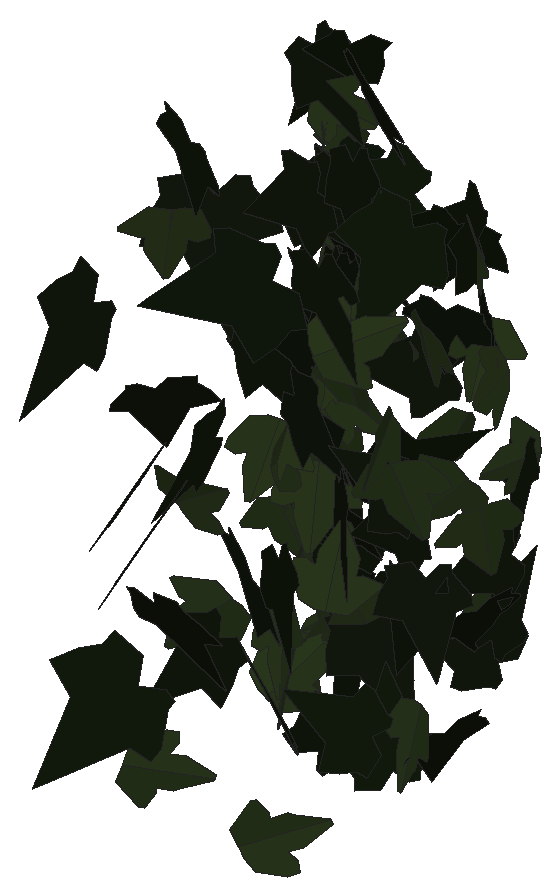
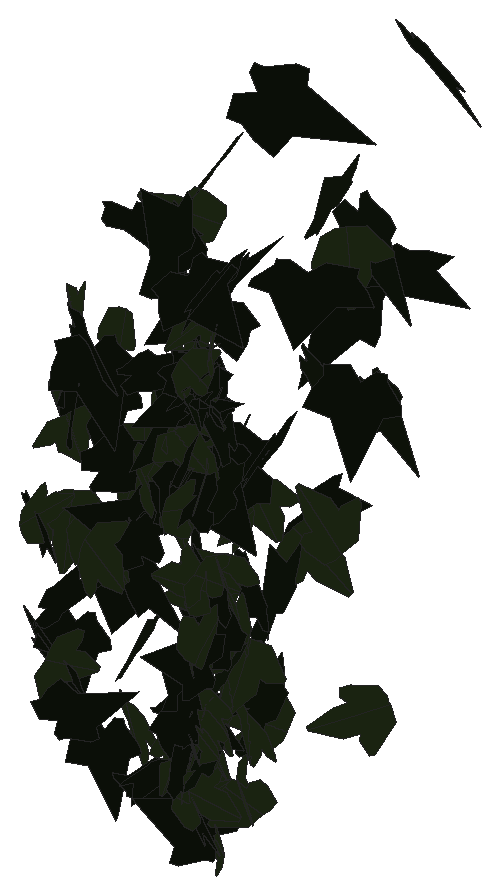
# SketchUp Ruby script. Lengths in inches.
U = 1.inch
M = Sketchup.active_model
def pt(a) = Geom::Point3d.new(a.map { |v| v * U })
def face(e, loops, mat)
  f = e.add_face(loops[0].map { |a| pt(a) })
  loops[1..].each { |l| e.add_face(l.map { |a| pt(a) }).erase! }
  f.material = f.back_material = mat if mat
  f
end
# faces: each face lists its corners as indices into pts; further lists are holes
def faces(e, pts, list, mat = nil) = list.each { |f| face(e, (f[0].is_a?(Array) ? f : [f]).map { |l| l.map { |i| pts[i] } }, mat) }
# xy, xz, yz: faces in a plane at the given z, y or x. An outline is a flat list of corners, or four numbers for a rectangle; further outlines are holes
def ring(l) = l.size == 4 ? [[l[0], l[1]], [l[2], l[1]], [l[2], l[3]], [l[0], l[3]]] : l.each_slice(2).to_a
def flat(e, list, mat, &to3) = list.each { |f| face(e, (f[0].is_a?(Array) ? f : [f]).map { |l| ring(l).map { |u, v| to3.(u, v) } }, mat) }
def xy(e, z, list, mat = nil) = flat(e, list, mat) { |x, y| [x, y, z] }
def xz(e, y, list, mat = nil) = flat(e, list, mat) { |x, z| [x, y, z] }
def yz(e, x, list, mat = nil) = flat(e, list, mat) { |y, z| [x, y, z] }
def lines(e, pts, list) = list.each { |a, b| e.add_line(pt(pts[a]), pt(pts[b])) }
# prism: a flat outline (further loops are holes) pulled along v
def prism(e, loops, v, mat = nil)
  f = face(e, loops, mat); d = Geom::Vector3d.new(v.map { |x| x * U })
  f.pushpull(f.normal.samedirection?(d) ? d.length : -d.length)
end
def box(e, o, s, mat = nil) = prism(e, [[o, [o[0] + s[0], o[1], o[2]], [o[0] + s[0], o[1] + s[1], o[2]], [o[0], o[1] + s[1], o[2]]]], [0, 0, s[2]], mat)
def at(x, y, z, deg = 0) = Geom::Transformation.translation(pt([x, y, z])) * Geom::Transformation.rotation(ORIGIN, Z_AXIS, deg.degrees)
def axes(o, x, y, z) = Geom::Transformation.new([*x, 0, *y, 0, *z, 0, *pt(o).to_a, 1])
def part(name) = M.definitions.add(name)
# library, detail: a bought-in or finely detailed component or shape, given as its bounding box
def library(name, o, s) = part(name).tap { |d| box(d.entities, o, s) }
def detail(e, o, s) = box(e.add_group.entities, o, s)
def put(e, d, t, mat = nil) = e.add_instance(d, t).tap { |i| i.material = mat if mat }
def group(e, t, mat = nil) = e.add_group.tap { |g| g.transformation = t; g.material = mat if mat }.entities
root = M.entities
M.materials.add("efeu1").color = [18, 25, 13]
M.materials.add("efeu2").color = [43, 57, 29]
c1 = part("ivyleaf_9")
p = [[1.54,2.16,1.25],[1.36,2.04,1.19],[-0.21,0.99,0.68],[-0.71,1.11,0.82],[-0.85,0.86,0.67],[-0.8,0.17,0.21],
  [-0.9,-0.01,0.1],[-0.67,-0.16,-0.02],[-0.08,-0.08,-0.05],[-0.03,-0.6,-0.4],[0.65,-0.88,-0.66],[0.83,-0.6,-0.49],
  [1.29,-0.42,-0.43],[1.8125,-0.07,-0.26],[1.21,0.44,0.15]]
faces(c1.entities,p,[[0,1,2,3,4,5,6,7,8,9,10,11,12,13,14]],"efeu1")
c2 = part("ivyleaf_10")
p = [[0,0.5,-0.03],[-0.0625,2.02,-0.43],[-0.19,2.01,-0.46],[-0.54,1.05,-0.29],[-0.52,0.625,-0.18],[-0.83,0.76,-0.28],
  [-1.16,0.64,-0.33],[-1.15,0.33,-0.24],[-0.77,-0.39,0.02],[-0.3,-0.51,0.16],[0.04,-0.48,0.23],[-0.02,2.01,-0.4375],
  [-0.06,2.01,-0.43],[0.04,-0.49,0.23],[0.67,-0.49,0.14],[1.38,0.36,-0.2],[1.375,0.51,-0.24],[0.81,0.65,-0.19],
  [0.62,0.59,-0.15],[0.6,1.09,-0.28],[0.5,1.23,-0.31]]
faces(c2.entities,p,[[0,1,2,3,4,5,6,7,8,9,10],[11,12,0,13,14,15,16,17,18,19,20]],"efeu2")
put(root,c1,axes([593.49,106.23,195.84],[-1.19676,-0.85692,0.36484],[-0.30418,-0.20185,-1.47187],[0.88028,-1.23475,-0.01259]))
put(root,c1,axes([589.84,108.61,207.26],[-1.40402,0.10789,-0.47473],[0.46937,-0.0846,-1.40741],[-0.12921,-1.47969,0.04586]))
put(root,c1,axes([591.91,109.31,199.78],[-0.82844,1.1156,-0.43445],[0.25901,-0.3488,-1.38956],[-1.16885,-0.86799,0.00001]))
put(root,c1,axes([591.93,109.45,196.84],[1.36698,0.20054,-0.333],[-0.32963,-0.04725,-1.38161],[-0.20603,1.40616,0.00107]))
put(root,c1,axes([592.55,114.11,206.7],[-0.2824,-0.17863,-1.47318],[-0.89101,-1.17881,0.31374],[-1.1867,0.92759,0.11501]))
put(root,c1,axes([586.71,115.08,197.1],[-0.73872,0.86965,-0.39727],[0.23479,-0.32165,-1.14071],[-0.92681,-0.77464,0.02766]))
put(root,c1,axes([589.03,115.98,191.73],[0.11357,-0.29781,-1.14485],[0.41787,-1.06587,0.31872],[-1.10669,-0.43302,0.00285]))
put(root,c1,axes([588.2,116.8125,198.29],[-1.03044,0.56506,-0.40164],[0.33278,-0.22803,-1.17459],[-0.60816,-1.08219,0.03779]))
put(root,c1,axes([591.98,117.53,205.35],[0.5622,-1.14469,-0.00344],[-0.00106,0.00331,-1.2753],[1.14469,0.5622,0.0005]))
put(root,c2,axes([587.73,117.78,191.73],[-0.70045,-0.45354,0.88487],[-0.70763,-0.53302,-0.83335],[0.69854,-0.99474,0.0431]))
put(root,c2,axes([585.2,117.02,185.46],[-0.30594,-0.18891,-1.10884],[0.93562,0.59512,-0.35954],[0.62437,-0.98436,-0.00457]))
put(root,c2,axes([592.64,117.31,202.97],[0.47104,0.08984,-1.13989],[1.04532,0.46578,0.46867],[0.46339,-1.14205,0.10147]))
put(root,c1,axes([585.43,117.5,198.79],[0.55138,0.9579,-0.36912],[-0.18196,-0.32117,-1.10525],[-1.0103,0.58062,-0.00239]))
put(root,c2,axes([585.58,118.03,204.74],[-0.83319,-0.80668,0.12408],[-0.08924,-0.08621,-1.15972],[0.81128,-0.83795,-0.00014]))
put(root,c2,axes([589.29,117.74,183.75],[-0.31937,-0.3588,1.10004],[0.71901,0.83256,0.4803],[-0.90656,0.78672,-0.00659]))
put(root,c1,axes([585.32,119.29,206.875],[0.19106,-0.89981,0.77544],[0.26005,-0.73467,-0.91657],[1.15903,0.31317,0.07783]))
put(root,c2,axes([584.88,119.61,193.66],[-0.71816,-0.37332,0.86791],[0.90925,0.02311,0.76231],[-0.25671,1.12627,0.27204]))
put(root,c1,axes([586.5,120.95,190.82],[0.15345,-0.75568,1.20933],[0.37452,-1.15225,-0.76754],[1.37596,0.39791,0.07405]))
put(root,c1,axes([585.53,120.28,204.48],[-0.69526,-1.03479,-0.85927],[0.47215,0.71796,-1.24664],[1.25944,-0.8404,-0.00699]))
put(root,c1,axes([587.5,121.03,191.7],[-0.47974,-0.01407,-1.09963],[1.0994,0.02302,-0.47994],[0.02673,-1.1995,0.00368]))
put(root,c2,axes([590.47,120.92,198.96],[-1.07514,0.21259,-0.09072],[-0.09338,-0.0047,1.09573],[0.21144,1.07895,0.02264]))
put(root,c1,axes([586.43,121.67,186.62],[0.4031,-0.76021,1.06906],[0.51312,-0.93791,-0.86042],[1.20727,0.65246,0.00875]))
put(root,c1,axes([592.36,121.55,205.18],[-1.1912,-0.64338,-0.29041],[0.27205,0.10722,-1.35341],[0.65136,-1.22139,0.03416]))
put(root,c2,axes([591.42,121.68,197.65],[-0.13627,0.60985,-0.88681],[-0.02107,-0.89523,-0.6124],[-1.07606,-0.0597,0.12429]))
put(root,c2,axes([586.76,121.65,195.82],[0.99712,0.44571,-0.27095],[-0.25025,-0.10408,-1.09218],[-0.45765,1.02802,0.00689]))
put(root,c1,axes([587.49,122.8,204.3125],[0.35524,-0.81068,-0.76645],[0.31151,-0.70029,0.88509],[-1.07126,-0.47246,0.00322]))
put(root,c2,axes([591.79,121.73,196.09],[-1.08738,-0.54908,-0.30435],[0.28507,0.11046,-1.2178],[0.55933,-1.12375,0.029]))
put(root,c1,axes([587.72,121.68,197.45],[0.83063,-0.60092,-0.79642],[-0.61876,0.50265,-1.0246],[0.78264,1.03517,0.0352]))
put(root,c2,axes([588.91,121.8,190.88],[0.89299,0.65213,-0.2656],[0.19863,0.17823,1.10545],[0.67555,-0.91444,0.02605]))
put(root,c1,axes([589.97,122.42,185.84],[-0.65212,-0.58876,-0.57812],[-0.42585,-0.391,0.87857],[-0.70676,0.77884,0.00405]))
put(root,c1,axes([589.34,122.47,206.04],[-0.62706,-0.08927,-0.99726],[0.9845,0.15932,-0.6333],[0.18234,-1.16719,-0.01017]))
put(root,c1,axes([588.66,122.66,193.96],[-0.29492,0.05695,-1.17254],[1.15267,-0.21497,-0.30037],[-0.22238,-1.1898,-0.00186]))
put(root,c2,axes([587.04,121.84,194.93],[-0.01116,-0.01002,1.08265],[-0.42922,0.99404,0.00478],[-0.99399,-0.42913,-0.01422]))
put(root,c2,axes([592.35,122.46,201.06],[-0.9563,0.42967,0.2539],[-0.22828,0.11141,-1.04836],[-0.44381,-0.98314,-0.00783]))
put(root,c1,axes([585.34,122.53,198.77],[0.72175,-0.8285,-0.74715],[-0.45312,0.59548,-1.09802],[1.01947,0.85121,0.04092]))
put(root,c1,axes([590.43,123.63,194.08],[-0.08133,-1.06398,-0.14432],[-0.01093,-0.14391,1.06708],[-1.07367,0.08206,0.00006]))
put(root,c2,axes([590.93,123.51,186.16],[1.05007,-0.54064,0.06378],[0.06707,-0.00903,-1.18086],[0.54024,1.05197,0.02264]))
put(root,c2,axes([587.06,123.41,193.55],[1.08847,0.41556,0.02504],[0.02124,0.01456,-1.16508],[-0.41577,1.08866,0.00602]))
put(root,c1,axes([591.4,123.54,191.34],[-0.55953,-0.66645,-0.66208],[0.44583,0.48992,-0.86994],[0.82689,-0.71512,0.02103]))
put(root,c2,axes([585.41,123.68,187.79],[1.04298,-0.35063,0.45593],[0.43132,-0.14777,-1.10034],[0.38049,1.12865,-0.00242]))
put(root,c1,axes([587.07,123.4375,204.26],[-0.13523,-0.26499,-1.28924],[0.85725,0.9657,-0.28841],[0.99873,-0.86478,0.07299]))
put(root,c1,axes([589.875,124.63,189.53],[0.06857,-0.86871,0.80221],[0.10522,-0.79588,-0.87086],[1.17776,0.12168,0.03109]))
put(root,c1,axes([585.68,123.26,197.99],[0.31011,0.6953,-0.87256],[0.29199,0.82349,0.75997],[1.07682,-0.42353,0.04521]))
put(root,c2,axes([593.25,124.1,194.01],[-0.59791,-0.9866,-0.20442],[0.1185,0.1672,-1.15354],[1.00056,-0.60937,0.01446]))
put(root,c2,axes([584.99,124.68,185.79],[0.57578,-0.64484,0.59134],[0.42325,-0.41427,-0.86386],[0.76574,0.71385,0.03284]))
put(root,c2,axes([585.05,124.64,191.93],[-0.20049,0.06855,1.0293],[1.01584,-0.16936,0.20914],[0.17953,1.03488,-0.03396]))
put(root,c1,axes([590.08,124.44,192.66],[-0.03975,-0.04223,-1.10854],[-1.04483,-0.37134,0.05161],[-0.3728,1.04525,-0.02645]))
put(root,c1,axes([589.41,124.34,183.67],[-1.10272,-0.07093,0.2202],[0.21989,0.01182,1.105],[-0.07187,1.12443,0.00227]))
put(root,c1,axes([591.51,124.4,185.53],[-0.02435,1.0361,-0.24756],[0.00781,-0.24744,-1.03639],[-1.06524,-0.0255,-0.00194]))
put(root,c1,axes([589.47,124.12,194.27],[0.2514,0.03542,1.19047],[1.10025,0.45893,-0.246],[-0.45599,1.12686,0.06277]))
put(root,c1,axes([587.43,125.41,206.92],[0.91675,-0.21398,-1.13739],[1.13235,-0.13405,0.93791],[-0.2392,-1.45469,0.08088]))
put(root,c2,axes([584.8,124.77,191.23],[-0.93472,-0.62216,-0.26632],[0.22162,0.14768,-1.12285],[0.63945,-0.96063,-0.00013]))
put(root,c2,axes([591.57,125.05,194.23],[-0.78081,-0.29671,0.77164],[-0.72361,-0.26803,-0.83527],[0.39982,-1.06454,-0.00477]))
put(root,c2,axes([591.9375,125.42,202.62],[-0.23936,0.03101,0.97762],[0.85798,-0.47662,0.22519],[0.46966,0.88649,0.08688]))
put(root,c2,axes([593.3,124.83,198.84],[0.68694,-0.61217,-0.63555],[-0.48796,0.40754,-0.91998],[0.73523,0.84245,-0.01677]))
put(root,c2,axes([584.75,124.52,184.95],[0.75093,0.30671,-0.81484],[0.70132,0.42455,0.80612],[0.51593,-1.02353,0.0902]))
put(root,c1,axes([586.48,124.5,183.27],[-0.01661,-0.00892,1.2084],[1.0982,0.50417,0.01882],[-0.50425,1.09832,0.00117]))
put(root,c1,axes([591.0625,125.01,200.28],[0.69375,0.55576,-0.65751],[-0.50777,-0.41777,-0.88888],[-0.69524,0.8597,-0.0069]))
put(root,c1,axes([586.55,125.7,200.03],[-0.2727,0.53975,-0.86231],[0.37831,-0.77493,-0.60469],[-0.94435,-0.46631,0.00677]))
put(root,c1,axes([590.16,126.13,197.5],[-0.39443,-0.21627,1.14235],[-0.98738,-0.57459,-0.4497],[0.61385,-1.06319,0.01067]))
put(root,c2,axes([584.74,126.09,189.41],[-0.01139,0.14567,-0.94079],[0.13057,-0.93172,-0.14585],[-0.943,-0.13077,-0.00883]))
put(root,c1,axes([592.32,125.04,189.95],[0.06389,1.04021,-0.14729],[-0.01487,-0.14665,-1.04216],[-1.05049,0.06535,0.0058]))
put(root,c1,axes([585.16,125.93,193.2],[-0.03702,0.04644,1.00377],[0.48081,-0.88118,0.0585],[0.88235,0.48213,0.01023]))
put(root,c1,axes([592.32,126.53,191.34],[-0.32038,-0.56043,0.90184],[-0.46489,-0.77287,-0.64544],[0.9546,-0.56447,-0.01166]))
put(root,c1,axes([586.03,126.03,199.09],[-0.20151,0.89306,-1.14575],[0.24072,-1.1202,-0.91549],[-1.4326,-0.31384,0.00734]))
put(root,c1,axes([584.57,125.97,191.24],[0.49604,-0.75819,0.10332],[0.0566,-0.08644,-0.90604],[0.7631,0.49926,0.00004]))
put(root,c1,axes([584.77,125.93,200.64],[-0.05883,0.9737,0.89653],[0.05962,-0.89455,0.97547],[1.32224,0.08366,-0.0041]))
put(root,c1,axes([586.55,125.57,200.96],[1.14611,-0.0548,-0.0431],[-0.04225,0.01862,-1.1473],[0.05546,1.14677,0.01657]))
put(root,c1,axes([585.28,126.76,189.19],[0.43016,-0.37958,-1.19069],[1.07963,-0.52139,0.55625],[-0.62946,-1.15366,0.14037]))
put(root,c2,axes([587.76,126.35,197.65],[-0.43338,0.04636,1.15791],[1.09845,-0.37742,0.42623],[0.3692,1.17734,0.09105]))
put(root,c2,axes([584.63,125.98,193.96],[0.88153,-0.38874,-0.11752],[0.11305,-0.03487,0.96334],[-0.39006,-0.88865,0.01361]))
put(root,c1,axes([584.44,126.24,192.26],[0.2344,-0.13314,0.82645],[0.68107,-0.46866,-0.26867],[0.48671,0.71994,-0.02206]))
put(root,c2,axes([585.3,126.74,192.16],[-0.38629,-0.68739,-0.70041],[-0.33884,-0.61301,0.78848],[-0.92102,0.51382,0.00369]))
put(root,c2,axes([592.76,126.9,194.9],[-0.05304,0.11343,1.00782],[0.1271,-1.00049,0.1193],[1.00618,0.13236,0.03806]))
put(root,c2,axes([585.74,126.64,191.72],[0.1955,-0.26769,0.77723],[0.5936,-0.50669,-0.32382],[0.56867,0.62094,0.07083]))
put(root,c2,axes([585.43,126.45,199.21],[-0.45424,0.76289,-0.64453],[0.31103,-0.56479,-0.88771],[-0.94904,-0.55024,0.01756]))
put(root,c1,axes([584.99,126.06,207.16],[0.52746,-0.90498,-0.61778],[-0.29739,0.54166,-1.04739],[1.05461,0.60537,0.01363]))
put(root,c2,axes([584.83,126.69,204.26],[-0.1454,0.08747,0.86432],[0.65248,-0.56759,0.1672],[0.57356,0.66786,0.0289]))
put(root,c2,axes([586.86,126.4,198.76],[0.54822,0.08801,-1.01522],[-1.01038,-0.10295,-0.55453],[-0.1325,1.14919,0.02808]))
put(root,c2,axes([591.55,126.39,199.0625],[0.52703,0.85612,-0.31596],[-0.16276,-0.27083,-1.00533],[-0.89793,0.55158,-0.00321]))
put(root,c1,axes([586.91,126.44,186.91],[0.16448,-1.18494,-0.45824],[0.20717,0.4809,-1.16916],[1.25345,0.07601,0.25337]))
put(root,c2,axes([584.46,126.64,184.1875],[-0.0957,0.12222,-0.70869],[0.39524,-0.58834,-0.15484],[-0.6008,-0.40651,0.01103]))
put(root,c2,axes([586.68,126.02,187.65],[-0.46922,-0.78123,-0.43289],[0.21633,0.37502,-0.91128],[0.86655,-0.51664,-0.0069]))
put(root,c2,axes([585.43,126.76,186.49],[-0.3103,-0.90836,-0.4679],[-0.14445,-0.44509,0.95988],[-1.01152,0.34221,0.00646]))
put(root,c1,axes([592.12,125.92,198.84],[0.14754,-0.37544,1.02948],[-0.25015,0.9998,0.40047],[-1.06687,-0.28634,0.04847]))
put(root,c2,axes([585.13,126.79,195.21],[0.30553,0.47721,-0.73481],[-0.39564,-0.61921,-0.56664],[-0.78176,0.49988,-0.00041]))
put(root,c1,axes([584.14,126.44,198.89],[0.6814,-0.43292,0.32826],[0.27486,-0.17949,-0.80729],[0.46864,0.73474,-0.0038]))
put(root,c1,axes([592.13,126.06,188.62],[-0.69578,0.67658,0.54301],[0.3905,-0.37732,0.9705],[0.77468,0.79787,-0.0015]))
put(root,c1,axes([591.46,126.01,202.67],[-0.38846,0.05518,-1.16046],[-1.16177,-0.01654,0.38811],[0.00181,1.22364,0.05758]))
put(root,c1,axes([585.41,127.03,201.875],[-0.36772,-0.45338,0.54942],[-0.34155,-0.43038,-0.58374],[0.62511,-0.50185,0.00425]))
put(root,c2,axes([585.72,126.92,186.45],[0.015,0.01526,-0.78525],[-0.52658,-0.58252,-0.02138],[-0.58272,0.52679,-0.0009]))
put(root,c2,axes([589.8,127.09,194.75],[0.05505,-1.00057,0.68235],[0.1564,-0.67147,-0.99722],[1.20095,0.13331,0.09859]))
put(root,c1,axes([587.94,127.08,202.58],[-0.33178,-0.86753,-0.57155],[-0.19427,-0.5376,0.92877],[-1.02056,0.38436,0.00901]))
put(root,c1,axes([591.54,126.82,187.16],[-0.15318,0.01192,1.03275],[-1.02881,-0.09368,-0.15152],[0.09093,-1.03984,0.02549]))
put(root,c1,axes([585.68,126.8,207.16],[-0.02132,0.61343,-0.9605],[-0.01111,-0.96073,-0.61333],[-1.13961,-0.00211,0.02395]))
put(root,c1,axes([592.73,126.79,195.07],[-0.61903,0.01098,-0.81012],[0.80914,-0.0437,-0.61887],[-0.04138,-1.01862,0.01782]))
put(root,c1,axes([585.44,126.81,202.91],[0.09349,-0.89102,-0.09411],[-0.00651,0.09394,-0.8959],[0.89595,0.09366,0.00331]))
put(root,c1,axes([584.82,126.85,202.57],[0.56788,-0.10811,-0.63947],[0.63547,-0.07707,0.57735],[-0.12958,-0.85175,0.02892]))
put(root,c2,axes([591.5625,127.14,189.71],[0.27048,0.54148,-0.94122],[-0.40719,-0.84862,-0.60522],[-1.00663,0.48877,-0.00809]))
put(root,c1,axes([585.61,127.19,199.93],[0.20891,-0.26385,-0.75529],[0.49615,-0.56965,0.33623],[-0.62762,-0.53815,0.0144]))
put(root,c1,axes([585.56,125.67,202.11],[0.56545,0.56557,0.84246],[0.59593,0.59548,-0.79975],[-0.82126,0.82151,-0.00028]))
put(root,c2,axes([585.65,126.78,188.47],[0.51261,-0.61587,0.1522],[0.09663,-0.11759,-0.80129],[0.62699,0.52164,-0.00095]))
put(root,c1,axes([585.76,126.75,190.0625],[0.66142,-0.00563,-0.50493],[0.50198,0.09767,0.65646],[0.05482,-0.82638,0.08102]))
put(root,c2,axes([585.29,126.61,189.96],[0.89425,-0.25292,-0.49929],[-0.48035,0.1362,-0.92933],[0.28727,1.0151,0.00029]))
put(root,c2,axes([585.99,126.89,200.02],[0.34554,0.46132,0.68572],[-0.40474,-0.55356,0.57636],[0.72057,-0.53215,-0.0051]))
put(root,c2,axes([585.47,126.67,194.59],[0.16522,-0.01357,1.13543],[1.13183,0.09424,-0.16357],[-0.09132,1.14351,0.02695]))
put(root,c2,axes([585.5,126.01,205.44],[0.24798,0.45449,0.81369],[0.2272,0.78712,-0.50889],[-0.9039,0.32253,0.09532]))
put(root,c1,axes([584.875,127.14,187.58],[0.75002,-0.41565,-0.30233],[0.2639,-0.14752,0.8575],[-0.44105,-0.7951,-0.00105]))
put(root,c2,axes([585.36,127.17,186.45],[-0.26709,-0.43301,0.86468],[-0.45277,-0.73666,-0.50875],[0.8545,-0.52567,0.0007]))
put(root,c1,axes([586.42,126.24,185.74],[-0.4277,0.01596,-1.11731],[-1.11528,0.06797,0.4279],[0.06918,1.19445,-0.00942]))
put(root,c1,axes([585.63,126.83,202.41],[-0.66382,0.36994,-0.42007],[0.36256,-0.2123,-0.7599],[-0.42646,-0.75633,0.00784]))
put(root,c1,axes([586.01,127.12,198.61],[0.22339,-0.64276,0.39449],[0.13321,-0.37134,-0.68046],[0.74231,0.26007,0.00339]))
put(root,c1,axes([585.61,127.35,186.78],[0.08319,0.21624,1.08061],[-0.36963,-1.01543,0.23165],[1.03819,-0.37885,-0.00411]))
put(root,c1,axes([585.49,126.94,202.27],[-0.55855,-0.31313,-0.48717],[0.46689,0.15698,-0.63619],[0.34265,-0.72434,0.07273]))
put(root,c1,axes([585.01,126.74,191.66],[0.69657,-0.32613,0.64672],[0.59906,-0.2449,-0.76874],[0.4071,0.91841,0.02466]))
put(root,c2,axes([585.25,126.68,189.14],[0.83254,-0.39451,-0.53007],[-0.48004,0.22481,-0.92128],[0.45407,0.96102,-0.00209]))
put(root,c2,axes([585.48,127.11,203.75],[-0.20676,-0.65145,0.50513],[-0.14419,-0.48417,-0.68343],[0.81164,-0.25196,0.00726]))
put(root,c1,axes([590.27,126.57,202.39],[0.58625,0.58152,-0.87248],[-0.64231,-0.59091,-0.82544],[-0.82875,0.86934,0.02256]))
put(root,c2,axes([585.86,127,200.66],[0.82327,0.45347,-0.51906],[-0.46176,-0.23741,-0.93981],[-0.51169,0.94384,0.01299]))
put(root,c1,axes([585.74,127.3,189.69],[-0.06028,0.18485,-0.97603],[-0.07204,-0.97606,-0.18041],[-0.99076,0.05972,0.0725]))
put(root,c1,axes([585.55,126.46,203.22],[-0.09091,-0.39601,-0.88042],[0.14042,0.86948,-0.40559],[0.95511,-0.16553,-0.02417]))
put(root,c1,axes([585.48,127.13,197.74],[0.79404,0.10508,0.62208],[-0.61659,-0.08248,0.80096],[0.13358,-1.00533,-0.00069]))
put(root,c2,axes([585.76,127.55,197.96],[-0.10037,-0.09697,0.9298],[-0.08727,-0.93009,-0.10642],[0.93076,-0.09767,0.09029]))
put(root,c2,axes([586.05,126.98,197.92],[-0.30408,-0.72274,0.02966],[-0.01348,-0.02651,-0.7841],[0.72322,-0.30437,-0.00214]))
put(root,c2,axes([584.48,127.11,188.43],[0.23531,-0.14977,-0.68817],[0.59968,-0.33786,0.27859],[-0.36931,-0.64405,0.01389]))
